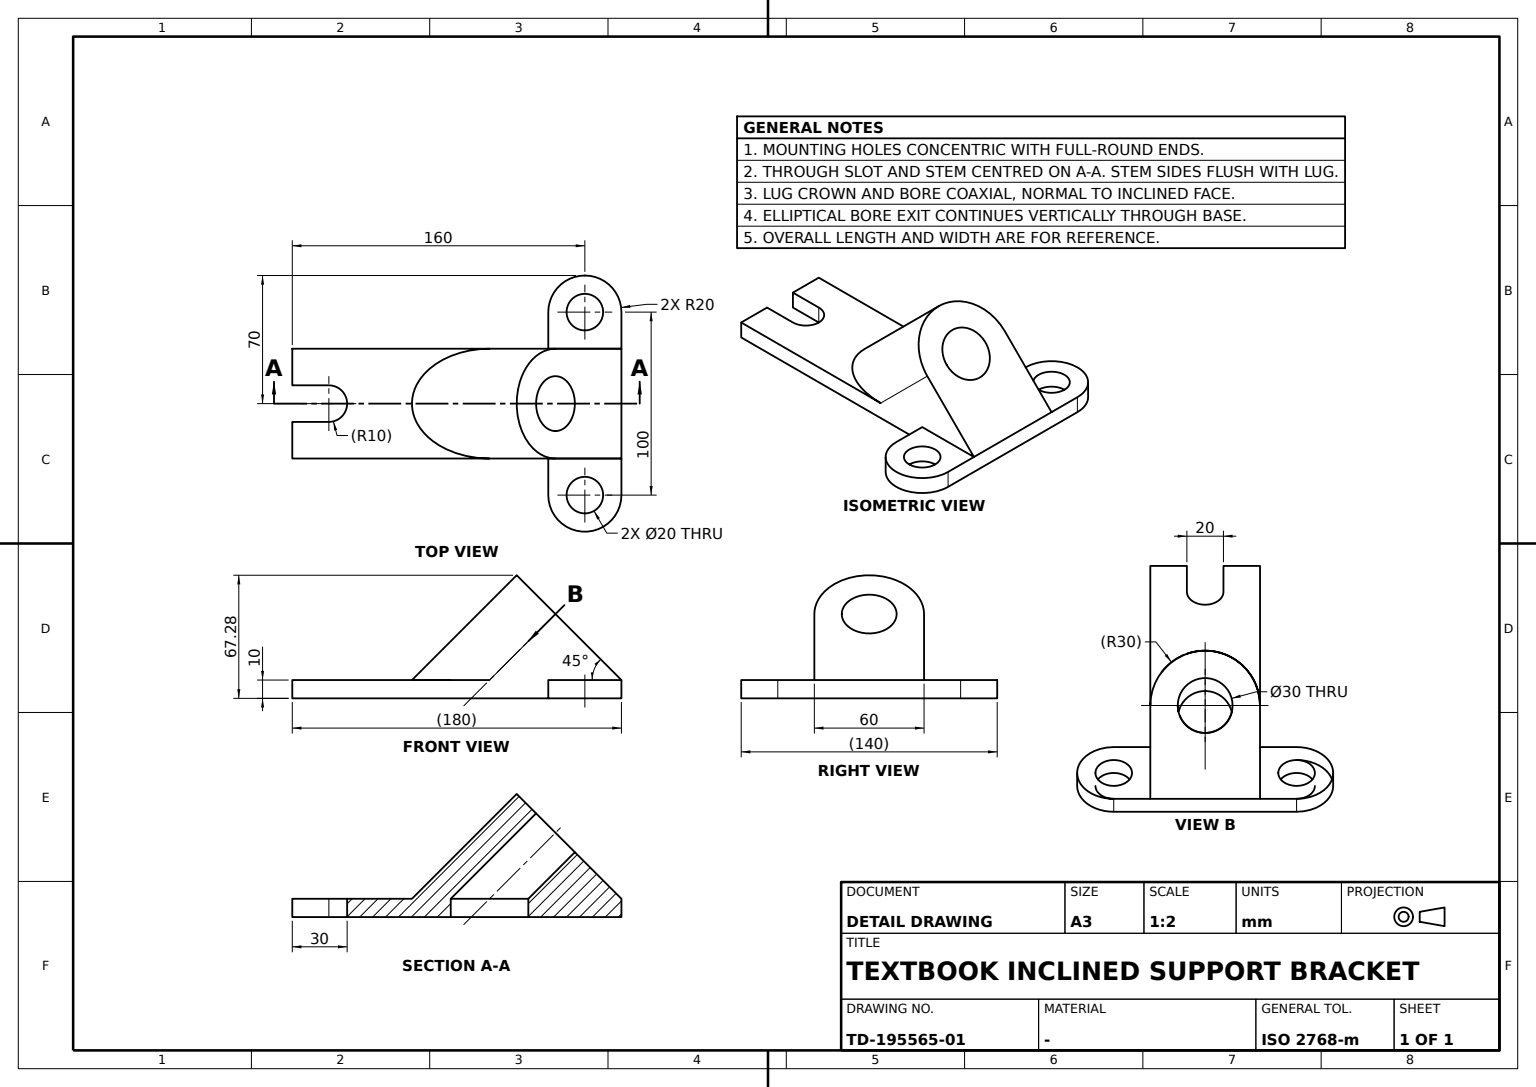
ISO-10303-21;
HEADER;
FILE_DESCRIPTION((''),'2;1');
FILE_NAME('','',(''),(''),'','','');
FILE_SCHEMA(('AUTOMOTIVE_DESIGN'));
ENDSEC;
DATA;
#1=APPLICATION_CONTEXT('');
#2=PRODUCT_CONTEXT('',#1,'mechanical');
#3=PRODUCT('','','',(#2));
#4=PRODUCT_DEFINITION_FORMATION('','',#3);
#5=PRODUCT_DEFINITION_CONTEXT('',#1,'design');
#6=PRODUCT_DEFINITION('','',#4,#5);
#7=PRODUCT_DEFINITION_SHAPE('','',#6);
#8=(LENGTH_UNIT()NAMED_UNIT(*)SI_UNIT(.MILLI.,.METRE.));
#9=(NAMED_UNIT(*)PLANE_ANGLE_UNIT()SI_UNIT($,.RADIAN.));
#10=(NAMED_UNIT(*)SI_UNIT($,.STERADIAN.)SOLID_ANGLE_UNIT());
#11=UNCERTAINTY_MEASURE_WITH_UNIT(LENGTH_MEASURE(1.E-05),#8,'distance_accuracy_value','');
#12=(GEOMETRIC_REPRESENTATION_CONTEXT(3)GLOBAL_UNCERTAINTY_ASSIGNED_CONTEXT((#11))GLOBAL_UNIT_ASSIGNED_CONTEXT((#8,#9,#10))REPRESENTATION_CONTEXT('',''));
#13=CARTESIAN_POINT('',(20.,50.,0.));
#14=VERTEX_POINT('',#13);
#15=CARTESIAN_POINT('',(20.,50.,-10.));
#16=VERTEX_POINT('',#15);
#17=CARTESIAN_POINT('',(20.,50.,-5.));
#18=DIRECTION('',(0.,0.,-1.));
#19=VECTOR('',#18,1000.);
#20=LINE('',#17,#19);
#21=EDGE_CURVE('',#14,#16,#20,.T.);
#22=ORIENTED_EDGE('',*,*,#21,.T.);
#23=CARTESIAN_POINT('',(0.,70.,-10.));
#24=VERTEX_POINT('',#23);
#25=CARTESIAN_POINT('',(0.,50.,-10.));
#26=DIRECTION('',(0.,0.,1.));
#27=DIRECTION('',(0.,1.,0.));
#28=AXIS2_PLACEMENT_3D('',#25,#26,#27);
#29=CIRCLE('',#28,20.);
#30=EDGE_CURVE('',#16,#24,#29,.T.);
#31=ORIENTED_EDGE('',*,*,#30,.T.);
#32=CARTESIAN_POINT('',(0.,70.,0.));
#33=VERTEX_POINT('',#32);
#34=CARTESIAN_POINT('',(0.,70.,-5.));
#35=LINE('',#34,#19);
#36=EDGE_CURVE('',#33,#24,#35,.T.);
#37=ORIENTED_EDGE('',*,*,#36,.F.);
#38=CARTESIAN_POINT('',(0.,50.,0.));
#39=AXIS2_PLACEMENT_3D('',#38,#26,#27);
#40=CIRCLE('',#39,20.);
#41=EDGE_CURVE('',#14,#33,#40,.T.);
#42=ORIENTED_EDGE('',*,*,#41,.F.);
#43=EDGE_LOOP('',(#22,#31,#37,#42));
#44=FACE_OUTER_BOUND('',#43,.T.);
#45=CARTESIAN_POINT('',(0.,50.,-5.));
#46=AXIS2_PLACEMENT_3D('',#45,#18,#27);
#47=CYLINDRICAL_SURFACE('',#46,20.);
#48=ADVANCED_FACE('',(#44),#47,.T.);
#49=ORIENTED_EDGE('',*,*,#36,.T.);
#50=CARTESIAN_POINT('',(-20.,50.,-10.));
#51=VERTEX_POINT('',#50);
#52=EDGE_CURVE('',#24,#51,#29,.T.);
#53=ORIENTED_EDGE('',*,*,#52,.T.);
#54=CARTESIAN_POINT('',(-20.,50.,0.));
#55=VERTEX_POINT('',#54);
#56=CARTESIAN_POINT('',(-20.,50.,-5.));
#57=LINE('',#56,#19);
#58=EDGE_CURVE('',#55,#51,#57,.T.);
#59=ORIENTED_EDGE('',*,*,#58,.F.);
#60=EDGE_CURVE('',#33,#55,#40,.T.);
#61=ORIENTED_EDGE('',*,*,#60,.F.);
#62=EDGE_LOOP('',(#49,#53,#59,#61));
#63=FACE_OUTER_BOUND('',#62,.T.);
#64=ADVANCED_FACE('',(#63),#47,.T.);
#65=CARTESIAN_POINT('',(-20.,-30.,0.));
#66=VERTEX_POINT('',#65);
#67=CARTESIAN_POINT('',(-20.,-50.,0.));
#68=VERTEX_POINT('',#67);
#69=CARTESIAN_POINT('',(-20.,-40.,0.));
#70=DIRECTION('',(0.,-1.,0.));
#71=VECTOR('',#70,1000.);
#72=LINE('',#69,#71);
#73=EDGE_CURVE('',#66,#68,#72,.T.);
#74=ORIENTED_EDGE('',*,*,#73,.F.);
#75=CARTESIAN_POINT('',(-20.,-30.,-10.));
#76=VERTEX_POINT('',#75);
#77=CARTESIAN_POINT('',(-20.,-30.,-5.));
#78=LINE('',#77,#19);
#79=EDGE_CURVE('',#66,#76,#78,.T.);
#80=ORIENTED_EDGE('',*,*,#79,.T.);
#81=CARTESIAN_POINT('',(-20.,-50.,-10.));
#82=VERTEX_POINT('',#81);
#83=CARTESIAN_POINT('',(-20.,-40.,-10.));
#84=LINE('',#83,#71);
#85=EDGE_CURVE('',#76,#82,#84,.T.);
#86=ORIENTED_EDGE('',*,*,#85,.T.);
#87=CARTESIAN_POINT('',(-20.,-50.,-5.));
#88=LINE('',#87,#19);
#89=EDGE_CURVE('',#68,#82,#88,.T.);
#90=ORIENTED_EDGE('',*,*,#89,.F.);
#91=EDGE_LOOP('',(#74,#80,#86,#90));
#92=FACE_OUTER_BOUND('',#91,.T.);
#93=CARTESIAN_POINT('',(-20.,30.,0.));
#94=DIRECTION('',(-1.,0.,0.));
#95=AXIS2_PLACEMENT_3D('',#93,#94,#27);
#96=PLANE('',#95);
#97=ADVANCED_FACE('',(#92),#96,.T.);
#98=CARTESIAN_POINT('',(0.,60.,-10.));
#99=VERTEX_POINT('',#98);
#100=CARTESIAN_POINT('',(0.,40.,-10.));
#101=VERTEX_POINT('',#100);
#102=CIRCLE('',#28,10.);
#103=EDGE_CURVE('',#99,#101,#102,.T.);
#104=ORIENTED_EDGE('',*,*,#103,.T.);
#105=EDGE_CURVE('',#101,#99,#102,.T.);
#106=ORIENTED_EDGE('',*,*,#105,.T.);
#107=EDGE_LOOP('',(#104,#106));
#108=FACE_BOUND('',#107,.T.);
#109=CARTESIAN_POINT('',(-52.1249,-15.,-10.));
#110=VERTEX_POINT('',#109);
#111=CARTESIAN_POINT('',(-52.124884,15.,-10.));
#112=VERTEX_POINT('',#111);
#113=CARTESIAN_POINT('',(-51.464255,-15.,-10.));
#114=CARTESIAN_POINT('',(-50.4775,-14.967538,-10.));
#115=CARTESIAN_POINT('',(-49.333657,-14.872855,-10.));
#116=CARTESIAN_POINT('',(-48.845018,-14.820103,-10.));
#117=CARTESIAN_POINT('',(-48.519609,-14.78223,-10.));
#118=CARTESIAN_POINT('',(-48.358208,-14.762091,-10.));
#119=CARTESIAN_POINT('',(-47.540806,-14.65313,-10.));
#120=CARTESIAN_POINT('',(-46.57273,-14.490561,-10.));
#121=CARTESIAN_POINT('',(-45.465718,-14.245219,-10.));
#122=CARTESIAN_POINT('',(-44.996087,-14.128141,-10.));
#123=CARTESIAN_POINT('',(-44.684066,-14.047437,-10.));
#124=CARTESIAN_POINT('',(-44.530553,-14.006305,-10.));
#125=CARTESIAN_POINT('',(-43.746021,-13.788565,-10.));
#126=CARTESIAN_POINT('',(-42.826179,-13.496945,-10.));
#127=CARTESIAN_POINT('',(-41.790825,-13.10364,-10.));
#128=CARTESIAN_POINT('',(-41.282596,-12.893718,-10.));
#129=CARTESIAN_POINT('',(-41.066809,-12.800907,-10.));
#130=CARTESIAN_POINT('',(-40.9234,-12.738402,-10.));
#131=CARTESIAN_POINT('',(-40.853165,-12.707389,-10.));
#132=CARTESIAN_POINT('',(-40.200687,-12.41542,-10.));
#133=CARTESIAN_POINT('',(-39.361148,-11.998288,-10.));
#134=CARTESIAN_POINT('',(-38.434944,-11.462915,-10.));
#135=CARTESIAN_POINT('',(-37.985157,-11.183048,-10.));
#136=CARTESIAN_POINT('',(-37.795243,-11.060495,-10.));
#137=CARTESIAN_POINT('',(-37.669269,-10.978213,-10.));
#138=CARTESIAN_POINT('',(-37.607907,-10.937658,-10.));
#139=CARTESIAN_POINT('',(-37.034946,-10.554288,-10.));
#140=CARTESIAN_POINT('',(-36.310126,-10.018991,-10.));
#141=CARTESIAN_POINT('',(-35.532976,-9.35224,-10.));
#142=CARTESIAN_POINT('',(-35.16152,-9.008305,-10.));
#143=CARTESIAN_POINT('',(-35.005993,-8.858641,-10.));
#144=CARTESIAN_POINT('',(-34.903123,-8.758363,-10.));
#145=CARTESIAN_POINT('',(-34.853167,-8.709044,-10.));
#146=CARTESIAN_POINT('',(-34.387949,-8.243621,-10.));
#147=CARTESIAN_POINT('',(-33.814771,-7.60411,-10.));
#148=CARTESIAN_POINT('',(-33.228508,-6.824857,-10.));
#149=CARTESIAN_POINT('',(-32.955987,-6.426941,-10.));
#150=CARTESIAN_POINT('',(-32.843609,-6.254629,-10.));
#151=CARTESIAN_POINT('',(-32.769672,-6.13936,-10.));
#152=CARTESIAN_POINT('',(-32.733816,-6.08253,-10.));
#153=CARTESIAN_POINT('',(-32.404339,-5.551247,-10.));
#154=CARTESIAN_POINT('',(-32.018446,-4.830623,-10.));
#155=CARTESIAN_POINT('',(-31.661704,-3.968463,-10.));
#156=CARTESIAN_POINT('',(-31.528842,-3.594373,-10.));
#157=CARTESIAN_POINT('',(-31.444719,-3.343959,-10.));
#158=CARTESIAN_POINT('',(-31.405233,-3.21942,-10.));
#159=CARTESIAN_POINT('',(-31.063576,-2.072772,-10.));
#160=CARTESIAN_POINT('',(-30.911717,-1.041455,-10.));
#161=CARTESIAN_POINT('',(-30.911684,0.521214,-10.));
#162=CARTESIAN_POINT('',(-30.968662,1.298476,-10.));
#163=CARTESIAN_POINT('',(-31.134877,2.198154,-10.));
#164=CARTESIAN_POINT('',(-31.227486,2.582202,-10.));
#165=CARTESIAN_POINT('',(-31.293974,2.837895,-10.));
#166=CARTESIAN_POINT('',(-31.330001,2.966942,-10.));
#167=CARTESIAN_POINT('',(-31.517929,3.59763,-10.));
#168=CARTESIAN_POINT('',(-31.796954,4.342448,-10.));
#169=CARTESIAN_POINT('',(-32.21613,5.190392,-10.));
#170=CARTESIAN_POINT('',(-32.449129,5.609112,-10.));
#171=CARTESIAN_POINT('',(-32.554002,5.787437,-10.));
#172=CARTESIAN_POINT('',(-32.625033,5.906071,-10.));
#173=CARTESIAN_POINT('',(-32.661773,5.966339,-10.));
#174=CARTESIAN_POINT('',(-32.985436,6.488252,-10.));
#175=CARTESIAN_POINT('',(-33.464246,7.165387,-10.));
#176=CARTESIAN_POINT('',(-34.105562,7.922569,-10.));
#177=CARTESIAN_POINT('',(-34.446896,8.292957,-10.));
#178=CARTESIAN_POINT('',(-34.597613,8.449938,-10.));
#179=CARTESIAN_POINT('',(-34.699075,8.554201,-10.));
#180=CARTESIAN_POINT('',(-34.75143,8.607269,-10.));
#181=CARTESIAN_POINT('',(-35.206692,9.062753,-10.));
#182=CARTESIAN_POINT('',(-35.85305,9.646104,-10.));
#183=CARTESIAN_POINT('',(-36.675981,10.284751,-10.));
#184=CARTESIAN_POINT('',(-37.104659,10.593591,-10.));
#185=CARTESIAN_POINT('',(-37.292066,10.723705,-10.));
#186=CARTESIAN_POINT('',(-37.417824,10.809948,-10.));
#187=CARTESIAN_POINT('',(-37.482477,10.853733,-10.));
#188=CARTESIAN_POINT('',(-38.043479,11.229116,-10.));
#189=CARTESIAN_POINT('',(-38.822157,11.701895,-10.));
#190=CARTESIAN_POINT('',(-39.784298,12.204942,-10.));
#191=CARTESIAN_POINT('',(-40.278789,12.444333,-10.));
#192=CARTESIAN_POINT('',(-40.49359,12.544329,-10.));
#193=CARTESIAN_POINT('',(-40.63743,12.610416,-10.));
#194=CARTESIAN_POINT('',(-40.711009,12.64377,-10.));
#195=CARTESIAN_POINT('',(-41.351977,12.930563,-10.));
#196=CARTESIAN_POINT('',(-42.228444,13.282712,-10.));
#197=CARTESIAN_POINT('',(-43.289218,13.640628,-10.));
#198=CARTESIAN_POINT('',(-43.829161,13.806355,-10.));
#199=CARTESIAN_POINT('',(-44.062613,13.874546,-10.));
#200=CARTESIAN_POINT('',(-44.218703,13.919377,-10.));
#201=CARTESIAN_POINT('',(-44.298075,13.941782,-10.));
#202=CARTESIAN_POINT('',(-44.994684,14.135104,-10.));
#203=CARTESIAN_POINT('',(-45.936536,14.361122,-10.));
#204=CARTESIAN_POINT('',(-47.058182,14.569257,-10.));
#205=CARTESIAN_POINT('',(-47.543777,14.646554,-10.));
#206=CARTESIAN_POINT('',(-47.868594,14.695439,-10.));
#207=CARTESIAN_POINT('',(-48.032751,14.71872,-10.));
#208=CARTESIAN_POINT('',(-49.493363,14.913453,-10.));
#209=CARTESIAN_POINT('',(-50.803311,14.999997,-10.));
#210=B_SPLINE_CURVE_WITH_KNOTS('',3,(#109,#113,#114,#115,#116,#117,#118,#119,#120,#121,#122,#123,#124,#125,#126,#127,#128,#129,#130,#131,#132,#133,#134,#135,#136,#137,#138,#139,#140,#141,#142,#143,#144,#145,#146,#147,#148,#149,#150,#151,#152,#153,#154,#155,#156,#157,#158,#159,#160,#161,#162,#163,#164,#165,#166,#167,#168,#169,#170,#171,#172,#173,#174,#175,#176,#177,#178,#179,#180,#181,#182,#183,#184,#185,#186,#187,#188,#189,#190,#191,#192,#193,#194,#195,#196,#197,#198,#199,#200,#201,#202,#203,#204,#205,#206,#207,#208,#209,#111),.UNSPECIFIED.,.F.,.F.,(4,1,1,2,2,1,1,2,2,1,1,1,2,2,1,1,1,2,2,1,1,1,2,2,1,1,1,2,2,1,1,2,2,2,1,1,2,2,1,1,1,2,2,1,1,1,2,2,1,1,1,2,2,1,1,1,2,2,1,1,1,2,2,1,1,2,2,4),(0.,0.03125,0.046875,0.0546875,0.0625,0.09375,0.109375,0.1171875,0.125,0.15625,0.171875,0.1796875,0.18359375,0.1875,0.21875,0.234375,0.2421875,0.24609375,0.25,0.28125,0.296875,0.3046875,0.30859375,0.3125,0.34375,0.359375,0.3671875,0.37109375,0.375,0.40625,0.421875,0.4296875,0.4375,0.5,0.53125,0.546875,0.5546875,0.5625,0.59375,0.609375,0.6171875,0.62109375,0.625,0.65625,0.671875,0.6796875,0.68359375,0.6875,0.71875,0.734375,0.7421875,0.74609375,0.75,0.78125,0.796875,0.8046875,0.80859375,0.8125,0.84375,0.859375,0.8671875,0.87109375,0.875,0.90625,0.921875,0.9296875,0.9375,1.),.UNSPECIFIED.);
#211=EDGE_CURVE('',#110,#112,#210,.T.);
#212=ORIENTED_EDGE('',*,*,#211,.T.);
#213=CARTESIAN_POINT('',(-52.785777,14.999988,-10.));
#214=CARTESIAN_POINT('',(-53.772897,14.9675,-10.));
#215=CARTESIAN_POINT('',(-54.753686,14.886288,-10.));
#216=CARTESIAN_POINT('',(-55.406139,14.821318,-10.));
#217=CARTESIAN_POINT('',(-55.729535,14.783704,-10.));
#218=CARTESIAN_POINT('',(-56.710377,14.652915,-10.));
#219=CARTESIAN_POINT('',(-57.678403,14.490313,-10.));
#220=CARTESIAN_POINT('',(-58.785341,14.244935,-10.));
#221=CARTESIAN_POINT('',(-59.254938,14.127843,-10.));
#222=CARTESIAN_POINT('',(-59.566935,14.04713,-10.));
#223=CARTESIAN_POINT('',(-59.720493,14.005977,-10.));
#224=CARTESIAN_POINT('',(-60.504673,13.788294,-10.));
#225=CARTESIAN_POINT('',(-61.424119,13.496763,-10.));
#226=CARTESIAN_POINT('',(-62.459062,13.103599,-10.));
#227=CARTESIAN_POINT('',(-62.967096,12.893755,-10.));
#228=CARTESIAN_POINT('',(-63.182803,12.80098,-10.));
#229=CARTESIAN_POINT('',(-63.326159,12.738499,-10.));
#230=CARTESIAN_POINT('',(-63.396345,12.70751,-10.));
#231=CARTESIAN_POINT('',(-64.048804,12.415558,-10.));
#232=CARTESIAN_POINT('',(-64.888319,11.998449,-10.));
#233=CARTESIAN_POINT('',(-65.814499,11.463106,-10.));
#234=CARTESIAN_POINT('',(-66.264276,11.183255,-10.));
#235=CARTESIAN_POINT('',(-66.454184,11.060708,-10.));
#236=CARTESIAN_POINT('',(-66.580156,10.978431,-10.));
#237=CARTESIAN_POINT('',(-66.641495,10.937892,-10.));
#238=CARTESIAN_POINT('',(-67.21463,10.554417,-10.));
#239=CARTESIAN_POINT('',(-67.93965,10.018983,-10.));
#240=CARTESIAN_POINT('',(-68.716978,9.352079,-10.));
#241=CARTESIAN_POINT('',(-69.088509,9.008068,-10.));
#242=CARTESIAN_POINT('',(-69.244066,8.858373,-10.));
#243=CARTESIAN_POINT('',(-69.346954,8.758073,-10.));
#244=CARTESIAN_POINT('',(-69.396928,8.708735,-10.));
#245=CARTESIAN_POINT('',(-69.86215,8.243291,-10.));
#246=CARTESIAN_POINT('',(-70.435334,7.603739,-10.));
#247=CARTESIAN_POINT('',(-71.021601,6.824415,-10.));
#248=CARTESIAN_POINT('',(-71.294123,6.426458,-10.));
#249=CARTESIAN_POINT('',(-71.406501,6.254128,-10.));
#250=CARTESIAN_POINT('',(-71.480438,6.138846,-10.));
#251=CARTESIAN_POINT('',(-71.516301,6.082001,-10.));
#252=CARTESIAN_POINT('',(-71.845728,5.550738,-10.));
#253=CARTESIAN_POINT('',(-72.23156,4.830146,-10.));
#254=CARTESIAN_POINT('',(-72.588241,3.96803,-10.));
#255=CARTESIAN_POINT('',(-72.721077,3.593961,-10.));
#256=CARTESIAN_POINT('',(-72.805184,3.343561,-10.));
#257=CARTESIAN_POINT('',(-72.844667,3.219014,-10.));
#258=CARTESIAN_POINT('',(-73.186211,2.072576,-10.));
#259=CARTESIAN_POINT('',(-73.338033,1.041624,-10.));
#260=CARTESIAN_POINT('',(-73.338106,-0.520967,-10.));
#261=CARTESIAN_POINT('',(-73.281152,-1.298191,-10.));
#262=CARTESIAN_POINT('',(-73.114973,-2.197829,-10.));
#263=CARTESIAN_POINT('',(-73.022382,-2.581862,-10.));
#264=CARTESIAN_POINT('',(-72.955905,-2.837544,-10.));
#265=CARTESIAN_POINT('',(-72.919887,-2.966577,-10.));
#266=CARTESIAN_POINT('',(-72.731976,-3.597282,-10.));
#267=CARTESIAN_POINT('',(-72.45297,-4.342121,-10.));
#268=CARTESIAN_POINT('',(-72.033814,-5.190088,-10.));
#269=CARTESIAN_POINT('',(-71.800823,-5.608818,-10.));
#270=CARTESIAN_POINT('',(-71.695953,-5.787148,-10.));
#271=CARTESIAN_POINT('',(-71.624925,-5.905785,-10.));
#272=CARTESIAN_POINT('',(-71.588186,-5.966055,-10.));
#273=CARTESIAN_POINT('',(-71.264534,-6.487978,-10.));
#274=CARTESIAN_POINT('',(-70.785736,-7.165129,-10.));
#275=CARTESIAN_POINT('',(-70.144428,-7.922333,-10.));
#276=CARTESIAN_POINT('',(-69.803096,-8.292733,-10.));
#277=CARTESIAN_POINT('',(-69.65238,-8.449719,-10.));
#278=CARTESIAN_POINT('',(-69.550919,-8.553985,-10.));
#279=CARTESIAN_POINT('',(-69.498564,-8.607055,-10.));
#280=CARTESIAN_POINT('',(-69.04331,-9.062548,-10.));
#281=CARTESIAN_POINT('',(-68.396962,-9.645911,-10.));
#282=CARTESIAN_POINT('',(-67.57404,-10.284571,-10.));
#283=CARTESIAN_POINT('',(-67.145367,-10.593418,-10.));
#284=CARTESIAN_POINT('',(-66.957962,-10.723535,-10.));
#285=CARTESIAN_POINT('',(-66.832205,-10.80978,-10.));
#286=CARTESIAN_POINT('',(-66.767551,-10.853567,-10.));
#287=CARTESIAN_POINT('',(-66.206564,-11.228953,-10.));
#288=CARTESIAN_POINT('',(-65.427906,-11.701736,-10.));
#289=CARTESIAN_POINT('',(-64.465789,-12.204789,-10.));
#290=CARTESIAN_POINT('',(-63.971311,-12.444183,-10.));
#291=CARTESIAN_POINT('',(-63.756516,-12.544181,-10.));
#292=CARTESIAN_POINT('',(-63.61268,-12.610269,-10.));
#293=CARTESIAN_POINT('',(-63.539104,-12.643623,-10.));
#294=CARTESIAN_POINT('',(-62.898138,-12.930427,-10.));
#295=CARTESIAN_POINT('',(-62.021669,-13.28259,-10.));
#296=CARTESIAN_POINT('',(-60.96089,-13.640524,-10.));
#297=CARTESIAN_POINT('',(-60.420942,-13.806259,-10.));
#298=CARTESIAN_POINT('',(-60.187487,-13.874454,-10.));
#299=CARTESIAN_POINT('',(-60.031396,-13.919286,-10.));
#300=CARTESIAN_POINT('',(-59.952025,-13.941692,-10.));
#301=CARTESIAN_POINT('',(-59.255395,-14.135029,-10.));
#302=CARTESIAN_POINT('',(-58.313513,-14.361064,-10.));
#303=CARTESIAN_POINT('',(-57.191829,-14.569217,-10.));
#304=CARTESIAN_POINT('',(-56.706218,-14.64652,-10.));
#305=CARTESIAN_POINT('',(-56.38139,-14.69541,-10.));
#306=CARTESIAN_POINT('',(-56.217229,-14.718693,-10.));
#307=CARTESIAN_POINT('',(-54.756558,-14.913444,-10.));
#308=CARTESIAN_POINT('',(-53.446547,-15.,-10.));
#309=B_SPLINE_CURVE_WITH_KNOTS('',3,(#111,#213,#214,#215,#216,#217,#218,#219,#220,#221,#222,#223,#224,#225,#226,#227,#228,#229,#230,#231,#232,#233,#234,#235,#236,#237,#238,#239,#240,#241,#242,#243,#244,#245,#246,#247,#248,#249,#250,#251,#252,#253,#254,#255,#256,#257,#258,#259,#260,#261,#262,#263,#264,#265,#266,#267,#268,#269,#270,#271,#272,#273,#274,#275,#276,#277,#278,#279,#280,#281,#282,#283,#284,#285,#286,#287,#288,#289,#290,#291,#292,#293,#294,#295,#296,#297,#298,#299,#300,#301,#302,#303,#304,#305,#306,#307,#308,#109),.UNSPECIFIED.,.F.,.F.,(4,1,2,2,1,1,2,2,1,1,1,2,2,1,1,1,2,2,1,1,1,2,2,1,1,1,2,2,1,1,2,2,2,1,1,2,2,1,1,1,2,2,1,1,1,2,2,1,1,1,2,2,1,1,1,2,2,1,1,1,2,2,1,1,2,2,4),(0.,0.03125,0.046875,0.0625,0.09375,0.109375,0.1171875,0.125,0.15625,0.171875,0.1796875,0.18359375,0.1875,0.21875,0.234375,0.2421875,0.24609375,0.25,0.28125,0.296875,0.3046875,0.30859375,0.3125,0.34375,0.359375,0.3671875,0.37109375,0.375,0.40625,0.421875,0.4296875,0.4375,0.5,0.53125,0.546875,0.5546875,0.5625,0.59375,0.609375,0.6171875,0.62109375,0.625,0.65625,0.671875,0.6796875,0.68359375,0.6875,0.71875,0.734375,0.7421875,0.74609375,0.75,0.78125,0.796875,0.8046875,0.80859375,0.8125,0.84375,0.859375,0.8671875,0.87109375,0.875,0.90625,0.921875,0.9296875,0.9375,1.),.UNSPECIFIED.);
#310=EDGE_CURVE('',#112,#110,#309,.T.);
#311=ORIENTED_EDGE('',*,*,#310,.T.);
#312=EDGE_LOOP('',(#212,#311));
#313=FACE_BOUND('',#312,.T.);
#314=CARTESIAN_POINT('',(0.,-60.,-10.));
#315=VERTEX_POINT('',#314);
#316=CARTESIAN_POINT('',(0.,-40.,-10.));
#317=VERTEX_POINT('',#316);
#318=CARTESIAN_POINT('',(0.,-50.,-10.));
#319=AXIS2_PLACEMENT_3D('',#318,#26,#27);
#320=CIRCLE('',#319,10.);
#321=EDGE_CURVE('',#315,#317,#320,.T.);
#322=ORIENTED_EDGE('',*,*,#321,.T.);
#323=EDGE_CURVE('',#317,#315,#320,.T.);
#324=ORIENTED_EDGE('',*,*,#323,.T.);
#325=EDGE_LOOP('',(#322,#324));
#326=FACE_BOUND('',#325,.T.);
#327=CARTESIAN_POINT('',(-20.,30.,-10.));
#328=VERTEX_POINT('',#327);
#329=CARTESIAN_POINT('',(-159.999708,30.,-10.));
#330=VERTEX_POINT('',#329);
#331=CARTESIAN_POINT('',(-89.999854,30.,-10.));
#332=VECTOR('',#94,1000.);
#333=LINE('',#331,#332);
#334=EDGE_CURVE('',#328,#330,#333,.T.);
#335=ORIENTED_EDGE('',*,*,#334,.F.);
#336=CARTESIAN_POINT('',(-20.,40.,-10.));
#337=LINE('',#336,#71);
#338=EDGE_CURVE('',#51,#328,#337,.T.);
#339=ORIENTED_EDGE('',*,*,#338,.F.);
#340=ORIENTED_EDGE('',*,*,#52,.F.);
#341=ORIENTED_EDGE('',*,*,#30,.F.);
#342=CARTESIAN_POINT('',(20.,-50.,-10.));
#343=VERTEX_POINT('',#342);
#344=CARTESIAN_POINT('',(20.,0.,-10.));
#345=VECTOR('',#27,1000.);
#346=LINE('',#344,#345);
#347=EDGE_CURVE('',#343,#16,#346,.T.);
#348=ORIENTED_EDGE('',*,*,#347,.F.);
#349=CIRCLE('',#319,20.);
#350=EDGE_CURVE('',#82,#343,#349,.T.);
#351=ORIENTED_EDGE('',*,*,#350,.F.);
#352=ORIENTED_EDGE('',*,*,#85,.F.);
#353=CARTESIAN_POINT('',(-159.999708,-30.,-10.));
#354=VERTEX_POINT('',#353);
#355=CARTESIAN_POINT('',(-89.999854,-30.,-10.));
#356=DIRECTION('',(1.,0.,0.));
#357=VECTOR('',#356,1000.);
#358=LINE('',#355,#357);
#359=EDGE_CURVE('',#354,#76,#358,.T.);
#360=ORIENTED_EDGE('',*,*,#359,.F.);
#361=CARTESIAN_POINT('',(-159.999708,-10.,-10.));
#362=VERTEX_POINT('',#361);
#363=CARTESIAN_POINT('',(-159.999708,-20.,-10.));
#364=LINE('',#363,#71);
#365=EDGE_CURVE('',#362,#354,#364,.T.);
#366=ORIENTED_EDGE('',*,*,#365,.F.);
#367=CARTESIAN_POINT('',(-139.999708,-10.,-10.));
#368=VERTEX_POINT('',#367);
#369=CARTESIAN_POINT('',(-149.999708,-10.,-10.));
#370=LINE('',#369,#357);
#371=EDGE_CURVE('',#362,#368,#370,.T.);
#372=ORIENTED_EDGE('',*,*,#371,.T.);
#373=CARTESIAN_POINT('',(-139.999708,10.,-10.));
#374=VERTEX_POINT('',#373);
#375=CARTESIAN_POINT('',(-139.999708,0.,-10.));
#376=AXIS2_PLACEMENT_3D('',#375,#26,#27);
#377=CIRCLE('',#376,10.);
#378=EDGE_CURVE('',#368,#374,#377,.T.);
#379=ORIENTED_EDGE('',*,*,#378,.T.);
#380=CARTESIAN_POINT('',(-159.999708,10.,-10.));
#381=VERTEX_POINT('',#380);
#382=CARTESIAN_POINT('',(-149.999708,10.,-10.));
#383=LINE('',#382,#332);
#384=EDGE_CURVE('',#374,#381,#383,.T.);
#385=ORIENTED_EDGE('',*,*,#384,.T.);
#386=CARTESIAN_POINT('',(-159.999708,20.,-10.));
#387=LINE('',#386,#71);
#388=EDGE_CURVE('',#330,#381,#387,.T.);
#389=ORIENTED_EDGE('',*,*,#388,.F.);
#390=EDGE_LOOP('',(#335,#339,#340,#341,#348,#351,#352,#360,#366,#372,#379,#385,#389));
#391=FACE_OUTER_BOUND('',#390,.T.);
#392=CARTESIAN_POINT('',(0.,0.,-10.));
#393=AXIS2_PLACEMENT_3D('',#392,#26,#27);
#394=PLANE('',#393);
#395=ADVANCED_FACE('',(#108,#313,#326,#391),#394,.F.);
#396=CARTESIAN_POINT('',(-139.999708,-10.,0.));
#397=VERTEX_POINT('',#396);
#398=CARTESIAN_POINT('',(-139.999708,-10.,-5.));
#399=LINE('',#398,#19);
#400=EDGE_CURVE('',#397,#368,#399,.T.);
#401=ORIENTED_EDGE('',*,*,#400,.F.);
#402=CARTESIAN_POINT('',(-139.999708,10.,0.));
#403=VERTEX_POINT('',#402);
#404=CARTESIAN_POINT('',(-139.999708,0.,0.));
#405=AXIS2_PLACEMENT_3D('',#404,#26,#27);
#406=CIRCLE('',#405,10.);
#407=EDGE_CURVE('',#397,#403,#406,.T.);
#408=ORIENTED_EDGE('',*,*,#407,.T.);
#409=CARTESIAN_POINT('',(-139.999708,10.,-5.));
#410=LINE('',#409,#19);
#411=EDGE_CURVE('',#403,#374,#410,.T.);
#412=ORIENTED_EDGE('',*,*,#411,.T.);
#413=ORIENTED_EDGE('',*,*,#378,.F.);
#414=EDGE_LOOP('',(#401,#408,#412,#413));
#415=FACE_OUTER_BOUND('',#414,.T.);
#416=CARTESIAN_POINT('',(-139.999708,0.,-5.));
#417=AXIS2_PLACEMENT_3D('',#416,#18,#27);
#418=CYLINDRICAL_SURFACE('',#417,10.);
#419=ADVANCED_FACE('',(#415),#418,.F.);
#420=CARTESIAN_POINT('',(-159.999708,-10.,0.));
#421=VERTEX_POINT('',#420);
#422=CARTESIAN_POINT('',(-149.999708,-10.,0.));
#423=LINE('',#422,#357);
#424=EDGE_CURVE('',#421,#397,#423,.T.);
#425=ORIENTED_EDGE('',*,*,#424,.F.);
#426=CARTESIAN_POINT('',(-159.999708,-30.,0.));
#427=VERTEX_POINT('',#426);
#428=CARTESIAN_POINT('',(-159.999708,-20.,0.));
#429=LINE('',#428,#71);
#430=EDGE_CURVE('',#421,#427,#429,.T.);
#431=ORIENTED_EDGE('',*,*,#430,.T.);
#432=CARTESIAN_POINT('',(-52.124892,-30.,0.));
#433=VERTEX_POINT('',#432);
#434=CARTESIAN_POINT('',(-106.0623,-30.,0.));
#435=LINE('',#434,#357);
#436=EDGE_CURVE('',#427,#433,#435,.T.);
#437=ORIENTED_EDGE('',*,*,#436,.T.);
#438=CARTESIAN_POINT('',(-52.124892,30.,0.));
#439=VERTEX_POINT('',#438);
#440=CARTESIAN_POINT('',(-55.125369,30.,0.));
#441=CARTESIAN_POINT('',(-58.125846,29.81244,0.));
#442=CARTESIAN_POINT('',(-61.110662,29.437321,0.));
#443=CARTESIAN_POINT('',(-66.743283,28.356856,0.));
#444=CARTESIAN_POINT('',(-72.184496,26.551422,0.));
#445=CARTESIAN_POINT('',(-74.713365,25.522769,0.));
#446=CARTESIAN_POINT('',(-79.216544,23.302689,0.));
#447=CARTESIAN_POINT('',(-83.340082,20.446852,0.));
#448=CARTESIAN_POINT('',(-85.124292,19.005473,0.));
#449=CARTESIAN_POINT('',(-87.94598,16.31053,0.));
#450=CARTESIAN_POINT('',(-90.300587,13.209992,0.));
#451=CARTESIAN_POINT('',(-91.179743,11.863508,0.));
#452=CARTESIAN_POINT('',(-92.638686,9.197936,0.));
#453=CARTESIAN_POINT('',(-93.663535,6.339541,0.));
#454=CARTESIAN_POINT('',(-94.039962,4.957233,0.));
#455=CARTESIAN_POINT('',(-94.551559,2.201809,0.));
#456=CARTESIAN_POINT('',(-94.609298,-0.599308,0.));
#457=CARTESIAN_POINT('',(-94.525967,-1.968667,0.));
#458=CARTESIAN_POINT('',(-94.154209,-4.583152,0.));
#459=CARTESIAN_POINT('',(-93.397722,-7.112102,0.));
#460=CARTESIAN_POINT('',(-92.94943,-8.300984,0.));
#461=CARTESIAN_POINT('',(-91.851529,-10.714644,0.));
#462=CARTESIAN_POINT('',(-90.448061,-12.965541,0.));
#463=CARTESIAN_POINT('',(-89.642449,-14.090338,0.));
#464=CARTESIAN_POINT('',(-87.057711,-17.280741,0.));
#465=CARTESIAN_POINT('',(-83.972737,-20.017792,0.));
#466=CARTESIAN_POINT('',(-81.763613,-21.632478,0.));
#467=CARTESIAN_POINT('',(-77.180091,-24.43313,0.));
#468=CARTESIAN_POINT('',(-72.234823,-26.527601,0.));
#469=CARTESIAN_POINT('',(-69.737963,-27.395842,0.));
#470=CARTESIAN_POINT('',(-64.766409,-28.788789,0.));
#471=CARTESIAN_POINT('',(-59.668925,-29.603805,0.));
#472=CARTESIAN_POINT('',(-57.160413,-29.867935,0.));
#473=CARTESIAN_POINT('',(-54.642652,-30.,0.));
#474=B_SPLINE_CURVE_WITH_KNOTS('',5,(#438,#440,#441,#442,#443,#444,#445,#446,#447,#448,#449,#450,#451,#452,#453,#454,#455,#456,#457,#458,#459,#460,#461,#462,#463,#464,#465,#466,#467,#468,#469,#470,#471,#472,#473,#432),.UNSPECIFIED.,.F.,.F.,(6,3,3,3,3,3,3,3,3,3,3,6),(0.,21.216579279,40.459374465,56.60389594,67.929780791,78.017290486,87.677943711,96.634362046,106.391148727,125.62394119,144.26592682,162.069183292),.UNSPECIFIED.);
#475=EDGE_CURVE('',#439,#433,#474,.T.);
#476=ORIENTED_EDGE('',*,*,#475,.F.);
#477=CARTESIAN_POINT('',(-159.999708,30.,0.));
#478=VERTEX_POINT('',#477);
#479=CARTESIAN_POINT('',(-106.0623,30.,0.));
#480=LINE('',#479,#332);
#481=EDGE_CURVE('',#439,#478,#480,.T.);
#482=ORIENTED_EDGE('',*,*,#481,.T.);
#483=CARTESIAN_POINT('',(-159.999708,10.,0.));
#484=VERTEX_POINT('',#483);
#485=CARTESIAN_POINT('',(-159.999708,20.,0.));
#486=LINE('',#485,#71);
#487=EDGE_CURVE('',#478,#484,#486,.T.);
#488=ORIENTED_EDGE('',*,*,#487,.T.);
#489=CARTESIAN_POINT('',(-149.999708,10.,0.));
#490=LINE('',#489,#332);
#491=EDGE_CURVE('',#403,#484,#490,.T.);
#492=ORIENTED_EDGE('',*,*,#491,.F.);
#493=ORIENTED_EDGE('',*,*,#407,.F.);
#494=EDGE_LOOP('',(#425,#431,#437,#476,#482,#488,#492,#493));
#495=FACE_OUTER_BOUND('',#494,.T.);
#496=CARTESIAN_POINT('',(0.,0.,0.));
#497=AXIS2_PLACEMENT_3D('',#496,#26,#27);
#498=PLANE('',#497);
#499=ADVANCED_FACE('',(#495),#498,.T.);
#500=ORIENTED_EDGE('',*,*,#424,.T.);
#501=ORIENTED_EDGE('',*,*,#400,.T.);
#502=ORIENTED_EDGE('',*,*,#371,.F.);
#503=CARTESIAN_POINT('',(-159.999708,-10.,-5.));
#504=LINE('',#503,#19);
#505=EDGE_CURVE('',#421,#362,#504,.T.);
#506=ORIENTED_EDGE('',*,*,#505,.F.);
#507=EDGE_LOOP('',(#500,#501,#502,#506));
#508=FACE_OUTER_BOUND('',#507,.T.);
#509=AXIS2_PLACEMENT_3D('',#396,#70,#94);
#510=PLANE('',#509);
#511=ADVANCED_FACE('',(#508),#510,.F.);
#512=CARTESIAN_POINT('',(-159.999708,10.,-5.));
#513=LINE('',#512,#19);
#514=EDGE_CURVE('',#484,#381,#513,.T.);
#515=ORIENTED_EDGE('',*,*,#514,.T.);
#516=ORIENTED_EDGE('',*,*,#384,.F.);
#517=ORIENTED_EDGE('',*,*,#411,.F.);
#518=ORIENTED_EDGE('',*,*,#491,.T.);
#519=EDGE_LOOP('',(#515,#516,#517,#518));
#520=FACE_OUTER_BOUND('',#519,.T.);
#521=AXIS2_PLACEMENT_3D('',#402,#70,#94);
#522=PLANE('',#521);
#523=ADVANCED_FACE('',(#520),#522,.T.);
#524=CARTESIAN_POINT('',(-16.062446,30.,36.062446));
#525=VERTEX_POINT('',#524);
#526=CARTESIAN_POINT('',(-16.062446,-30.,36.062446));
#527=VERTEX_POINT('',#526);
#528=CARTESIAN_POINT('',(-16.062446,0.,36.062446));
#529=DIRECTION('',(0.707106781,0.,0.707106781));
#530=AXIS2_PLACEMENT_3D('',#528,#529,#27);
#531=CIRCLE('',#530,30.);
#532=EDGE_CURVE('',#525,#527,#531,.T.);
#533=ORIENTED_EDGE('',*,*,#532,.T.);
#534=CARTESIAN_POINT('',(20.,-30.,0.));
#535=VERTEX_POINT('',#534);
#536=CARTESIAN_POINT('',(1.968777,-30.,18.031223));
#537=DIRECTION('',(0.707106781,0.,-0.707106781));
#538=VECTOR('',#537,1000.);
#539=LINE('',#536,#538);
#540=EDGE_CURVE('',#527,#535,#539,.T.);
#541=ORIENTED_EDGE('',*,*,#540,.T.);
#542=CARTESIAN_POINT('',(20.,30.,0.));
#543=VERTEX_POINT('',#542);
#544=CARTESIAN_POINT('',(20.,0.,0.));
#545=LINE('',#544,#345);
#546=EDGE_CURVE('',#535,#543,#545,.T.);
#547=ORIENTED_EDGE('',*,*,#546,.T.);
#548=CARTESIAN_POINT('',(1.968777,30.,18.031223));
#549=DIRECTION('',(-0.707106781,0.,0.707106781));
#550=VECTOR('',#549,1000.);
#551=LINE('',#548,#550);
#552=EDGE_CURVE('',#543,#525,#551,.T.);
#553=ORIENTED_EDGE('',*,*,#552,.T.);
#554=EDGE_LOOP('',(#533,#541,#547,#553));
#555=FACE_OUTER_BOUND('',#554,.T.);
#556=CARTESIAN_POINT('',(-16.062446,-15.,36.062446));
#557=VERTEX_POINT('',#556);
#558=CARTESIAN_POINT('',(-16.062446,15.,36.062446));
#559=VERTEX_POINT('',#558);
#560=CIRCLE('',#530,15.);
#561=EDGE_CURVE('',#557,#559,#560,.T.);
#562=ORIENTED_EDGE('',*,*,#561,.F.);
#563=EDGE_CURVE('',#559,#557,#560,.T.);
#564=ORIENTED_EDGE('',*,*,#563,.F.);
#565=EDGE_LOOP('',(#562,#564));
#566=FACE_BOUND('',#565,.T.);
#567=CARTESIAN_POINT('',(10.,0.,10.));
#568=AXIS2_PLACEMENT_3D('',#567,#529,#27);
#569=PLANE('',#568);
#570=ADVANCED_FACE('',(#555,#566),#569,.T.);
#571=ORIENTED_EDGE('',*,*,#323,.F.);
#572=CARTESIAN_POINT('',(0.,-40.,0.));
#573=VERTEX_POINT('',#572);
#574=CARTESIAN_POINT('',(0.,-40.,-5.));
#575=LINE('',#574,#19);
#576=EDGE_CURVE('',#573,#317,#575,.T.);
#577=ORIENTED_EDGE('',*,*,#576,.F.);
#578=CARTESIAN_POINT('',(0.,-60.,0.));
#579=VERTEX_POINT('',#578);
#580=CARTESIAN_POINT('',(0.,-50.,0.));
#581=AXIS2_PLACEMENT_3D('',#580,#26,#27);
#582=CIRCLE('',#581,10.);
#583=EDGE_CURVE('',#573,#579,#582,.T.);
#584=ORIENTED_EDGE('',*,*,#583,.T.);
#585=CARTESIAN_POINT('',(0.,-60.,-5.));
#586=LINE('',#585,#19);
#587=EDGE_CURVE('',#579,#315,#586,.T.);
#588=ORIENTED_EDGE('',*,*,#587,.T.);
#589=EDGE_LOOP('',(#571,#577,#584,#588));
#590=FACE_OUTER_BOUND('',#589,.T.);
#591=CARTESIAN_POINT('',(0.,-50.,-5.));
#592=AXIS2_PLACEMENT_3D('',#591,#18,#27);
#593=CYLINDRICAL_SURFACE('',#592,10.);
#594=ADVANCED_FACE('',(#590),#593,.F.);
#595=ORIENTED_EDGE('',*,*,#338,.T.);
#596=VERTEX_POINT('',#93);
#597=CARTESIAN_POINT('',(-20.,30.,-5.));
#598=LINE('',#597,#19);
#599=EDGE_CURVE('',#596,#328,#598,.T.);
#600=ORIENTED_EDGE('',*,*,#599,.F.);
#601=CARTESIAN_POINT('',(-20.,40.,0.));
#602=LINE('',#601,#71);
#603=EDGE_CURVE('',#55,#596,#602,.T.);
#604=ORIENTED_EDGE('',*,*,#603,.F.);
#605=ORIENTED_EDGE('',*,*,#58,.T.);
#606=EDGE_LOOP('',(#595,#600,#604,#605));
#607=FACE_OUTER_BOUND('',#606,.T.);
#608=ADVANCED_FACE('',(#607),#96,.T.);
#609=CARTESIAN_POINT('',(20.,40.,0.));
#610=LINE('',#609,#345);
#611=EDGE_CURVE('',#543,#14,#610,.T.);
#612=ORIENTED_EDGE('',*,*,#611,.F.);
#613=ORIENTED_EDGE('',*,*,#546,.F.);
#614=CARTESIAN_POINT('',(20.,-50.,0.));
#615=VERTEX_POINT('',#614);
#616=CARTESIAN_POINT('',(20.,-40.,0.));
#617=LINE('',#616,#345);
#618=EDGE_CURVE('',#615,#535,#617,.T.);
#619=ORIENTED_EDGE('',*,*,#618,.F.);
#620=CARTESIAN_POINT('',(20.,-50.,-5.));
#621=LINE('',#620,#19);
#622=EDGE_CURVE('',#615,#343,#621,.T.);
#623=ORIENTED_EDGE('',*,*,#622,.T.);
#624=ORIENTED_EDGE('',*,*,#347,.T.);
#625=ORIENTED_EDGE('',*,*,#21,.F.);
#626=EDGE_LOOP('',(#612,#613,#619,#623,#624,#625));
#627=FACE_OUTER_BOUND('',#626,.T.);
#628=AXIS2_PLACEMENT_3D('',#614,#94,#27);
#629=PLANE('',#628);
#630=ADVANCED_FACE('',(#627),#629,.F.);
#631=ORIENTED_EDGE('',*,*,#561,.T.);
#632=CARTESIAN_POINT('',(-52.124884,15.,0.));
#633=VERTEX_POINT('',#632);
#634=CARTESIAN_POINT('',(-92.713751,15.,-40.588859));
#635=DIRECTION('',(-0.707106781,0.,-0.707106781));
#636=VECTOR('',#635,1000.);
#637=LINE('',#634,#636);
#638=EDGE_CURVE('',#559,#633,#637,.T.);
#639=ORIENTED_EDGE('',*,*,#638,.T.);
#640=CARTESIAN_POINT('',(-52.1249,-15.,0.));
#641=VERTEX_POINT('',#640);
#642=CARTESIAN_POINT('',(-50.838065,-15.,-0.000006));
#643=CARTESIAN_POINT('',(-49.551235,-14.931003,-0.000007));
#644=CARTESIAN_POINT('',(-48.269336,-14.793008,0.));
#645=CARTESIAN_POINT('',(-45.685585,-14.370428,0.));
#646=CARTESIAN_POINT('',(-43.168286,-13.650025,0.));
#647=CARTESIAN_POINT('',(-41.914237,-13.205179,0.));
#648=CARTESIAN_POINT('',(-39.412527,-12.124713,0.));
#649=CARTESIAN_POINT('',(-37.101587,-10.679204,0.));
#650=CARTESIAN_POINT('',(-35.982532,-9.838201,0.));
#651=CARTESIAN_POINT('',(-34.277584,-8.272484,0.));
#652=CARTESIAN_POINT('',(-32.900452,-6.422509,0.));
#653=CARTESIAN_POINT('',(-32.416165,-5.647256,0.));
#654=CARTESIAN_POINT('',(-31.641245,-4.114253,0.));
#655=CARTESIAN_POINT('',(-31.156108,-2.468319,0.));
#656=CARTESIAN_POINT('',(-30.999315,-1.678779,0.));
#657=CARTESIAN_POINT('',(-30.838929,-0.103154,0.));
#658=CARTESIAN_POINT('',(-30.971523,1.474632,0.));
#659=CARTESIAN_POINT('',(-31.107968,2.242846,0.));
#660=CARTESIAN_POINT('',(-31.471639,3.586461,0.));
#661=CARTESIAN_POINT('',(-32.030195,4.85943,0.));
#662=CARTESIAN_POINT('',(-32.311116,5.403702,0.));
#663=CARTESIAN_POINT('',(-33.151821,6.819685,0.));
#664=CARTESIAN_POINT('',(-34.19775,8.097781,0.));
#665=CARTESIAN_POINT('',(-34.921242,8.842546,0.));
#666=CARTESIAN_POINT('',(-36.627755,10.351715,0.));
#667=CARTESIAN_POINT('',(-38.544784,11.586872,0.));
#668=CARTESIAN_POINT('',(-39.636925,12.181876,0.));
#669=CARTESIAN_POINT('',(-42.096245,13.316174,0.));
#670=CARTESIAN_POINT('',(-44.688001,14.109151,0.));
#671=CARTESIAN_POINT('',(-46.117175,14.443459,0.));
#672=CARTESIAN_POINT('',(-48.178327,14.789154,0.));
#673=CARTESIAN_POINT('',(-50.258657,14.951598,0.));
#674=CARTESIAN_POINT('',(-50.88036,14.983866,0.));
#675=CARTESIAN_POINT('',(-51.502622,15.,0.));
#676=B_SPLINE_CURVE_WITH_KNOTS('',5,(#640,#642,#643,#644,#645,#646,#647,#648,#649,#650,#651,#652,#653,#654,#655,#656,#657,#658,#659,#660,#661,#662,#663,#664,#665,#666,#667,#668,#669,#670,#671,#672,#673,#674,#675,#632),.UNSPECIFIED.,.F.,.F.,(6,3,3,3,3,3,3,3,3,3,3,6),(81.032552882,90.131857166,99.514673721,109.348402629,115.777327902,121.43816658,126.926738712,131.246583649,138.552902212,147.31689724,157.666651494,162.066705845),.UNSPECIFIED.);
#677=EDGE_CURVE('',#641,#633,#676,.T.);
#678=ORIENTED_EDGE('',*,*,#677,.F.);
#679=CARTESIAN_POINT('',(-92.713751,-15.,-40.588859));
#680=LINE('',#679,#636);
#681=EDGE_CURVE('',#557,#641,#680,.T.);
#682=ORIENTED_EDGE('',*,*,#681,.F.);
#683=EDGE_LOOP('',(#631,#639,#678,#682));
#684=FACE_OUTER_BOUND('',#683,.T.);
#685=CARTESIAN_POINT('',(-92.713751,0.,-40.588859));
#686=AXIS2_PLACEMENT_3D('',#685,#635,#27);
#687=CYLINDRICAL_SURFACE('',#686,15.);
#688=ADVANCED_FACE('',(#684),#687,.F.);
#689=ORIENTED_EDGE('',*,*,#321,.F.);
#690=ORIENTED_EDGE('',*,*,#587,.F.);
#691=EDGE_CURVE('',#579,#573,#582,.T.);
#692=ORIENTED_EDGE('',*,*,#691,.T.);
#693=ORIENTED_EDGE('',*,*,#576,.T.);
#694=EDGE_LOOP('',(#689,#690,#692,#693));
#695=FACE_OUTER_BOUND('',#694,.T.);
#696=ADVANCED_FACE('',(#695),#593,.F.);
#697=ORIENTED_EDGE('',*,*,#41,.T.);
#698=ORIENTED_EDGE('',*,*,#60,.T.);
#699=ORIENTED_EDGE('',*,*,#603,.T.);
#700=CARTESIAN_POINT('',(0.,30.,0.));
#701=LINE('',#700,#332);
#702=EDGE_CURVE('',#543,#596,#701,.T.);
#703=ORIENTED_EDGE('',*,*,#702,.F.);
#704=ORIENTED_EDGE('',*,*,#611,.T.);
#705=EDGE_LOOP('',(#697,#698,#699,#703,#704));
#706=FACE_OUTER_BOUND('',#705,.T.);
#707=CARTESIAN_POINT('',(0.,60.,0.));
#708=VERTEX_POINT('',#707);
#709=CARTESIAN_POINT('',(0.,40.,0.));
#710=VERTEX_POINT('',#709);
#711=CIRCLE('',#39,10.);
#712=EDGE_CURVE('',#708,#710,#711,.T.);
#713=ORIENTED_EDGE('',*,*,#712,.F.);
#714=EDGE_CURVE('',#710,#708,#711,.T.);
#715=ORIENTED_EDGE('',*,*,#714,.F.);
#716=EDGE_LOOP('',(#713,#715));
#717=FACE_BOUND('',#716,.T.);
#718=ADVANCED_FACE('',(#706,#717),#498,.T.);
#719=CARTESIAN_POINT('',(-73.338087,15.000006,0.));
#720=CARTESIAN_POINT('',(-83.944697,0.000008,0.));
#721=CARTESIAN_POINT('',(-73.338103,-14.999994,0.));
#722=(BOUNDED_CURVE()B_SPLINE_CURVE(4,(#632,#719,#720,#721,#640),.UNSPECIFIED.,.F.,.F.)B_SPLINE_CURVE_WITH_KNOTS((5,5),(122.431447342,204.052418733),.UNSPECIFIED.)CURVE()GEOMETRIC_REPRESENTATION_ITEM()RATIONAL_B_SPLINE_CURVE((1.,0.707106781,0.666666667,0.707106781,1.))REPRESENTATION_ITEM(''));
#723=EDGE_CURVE('',#633,#641,#722,.T.);
#724=ORIENTED_EDGE('',*,*,#723,.T.);
#725=CARTESIAN_POINT('',(-52.1249,-15.,-11.308158));
#726=LINE('',#725,#19);
#727=EDGE_CURVE('',#641,#110,#726,.T.);
#728=ORIENTED_EDGE('',*,*,#727,.T.);
#729=ORIENTED_EDGE('',*,*,#310,.F.);
#730=CARTESIAN_POINT('',(-52.124884,15.,-11.308158));
#731=LINE('',#730,#19);
#732=EDGE_CURVE('',#633,#112,#731,.T.);
#733=ORIENTED_EDGE('',*,*,#732,.F.);
#734=EDGE_LOOP('',(#724,#728,#729,#733));
#735=FACE_OUTER_BOUND('',#734,.T.);
#736=CARTESIAN_POINT('',(-73.338087,15.000006,-10.));
#737=CARTESIAN_POINT('',(-83.944697,0.000008,-10.));
#738=CARTESIAN_POINT('',(-73.338103,-14.999994,-10.));
#739=(BOUNDED_SURFACE()B_SPLINE_SURFACE(4,1,((#632,#111),(#719,#736),(#720,#737),(#721,#738),(#640,#109)),.UNSPECIFIED.,.F.,.F.,.F.)B_SPLINE_SURFACE_WITH_KNOTS((5,5),(2,2),(122.431447342,204.052418733),(0.,10.),.UNSPECIFIED.)GEOMETRIC_REPRESENTATION_ITEM()RATIONAL_B_SPLINE_SURFACE(((1.,1.),(0.707106781,0.707106781),(0.666666667,0.666666667),(0.707106781,0.707106781),(1.,1.)))REPRESENTATION_ITEM('')SURFACE());
#740=ADVANCED_FACE('',(#735),#739,.T.);
#741=ORIENTED_EDGE('',*,*,#727,.F.);
#742=ORIENTED_EDGE('',*,*,#677,.T.);
#743=ORIENTED_EDGE('',*,*,#732,.T.);
#744=ORIENTED_EDGE('',*,*,#211,.F.);
#745=EDGE_LOOP('',(#741,#742,#743,#744));
#746=FACE_OUTER_BOUND('',#745,.T.);
#747=CARTESIAN_POINT('',(-30.911696,-15.000006,0.));
#748=CARTESIAN_POINT('',(-30.911696,-15.000006,-10.));
#749=CARTESIAN_POINT('',(-20.305087,-0.000008,0.));
#750=CARTESIAN_POINT('',(-20.305087,-0.000008,-10.));
#751=CARTESIAN_POINT('',(-30.91168,14.999994,0.));
#752=CARTESIAN_POINT('',(-30.91168,14.999994,-10.));
#753=(BOUNDED_SURFACE()B_SPLINE_SURFACE(4,1,((#640,#109),(#747,#748),(#749,#750),(#751,#752),(#632,#111)),.UNSPECIFIED.,.F.,.F.,.F.)B_SPLINE_SURFACE_WITH_KNOTS((5,5),(2,2),(40.810475952,122.431447343),(0.,10.),.UNSPECIFIED.)GEOMETRIC_REPRESENTATION_ITEM()RATIONAL_B_SPLINE_SURFACE(((1.,1.),(0.707106781,0.707106781),(0.666666667,0.666666667),(0.707106781,0.707106781),(1.,1.)))REPRESENTATION_ITEM('')SURFACE());
#754=ADVANCED_FACE('',(#746),#753,.T.);
#755=CARTESIAN_POINT('',(0.,40.,-5.));
#756=LINE('',#755,#19);
#757=EDGE_CURVE('',#710,#101,#756,.T.);
#758=ORIENTED_EDGE('',*,*,#757,.F.);
#759=ORIENTED_EDGE('',*,*,#714,.T.);
#760=CARTESIAN_POINT('',(0.,60.,-5.));
#761=LINE('',#760,#19);
#762=EDGE_CURVE('',#708,#99,#761,.T.);
#763=ORIENTED_EDGE('',*,*,#762,.T.);
#764=ORIENTED_EDGE('',*,*,#105,.F.);
#765=EDGE_LOOP('',(#758,#759,#763,#764));
#766=FACE_OUTER_BOUND('',#765,.T.);
#767=CYLINDRICAL_SURFACE('',#46,10.);
#768=ADVANCED_FACE('',(#766),#767,.F.);
#769=CARTESIAN_POINT('',(-92.713751,30.,-40.588859));
#770=LINE('',#769,#636);
#771=EDGE_CURVE('',#525,#439,#770,.T.);
#772=ORIENTED_EDGE('',*,*,#771,.T.);
#773=ORIENTED_EDGE('',*,*,#475,.T.);
#774=CARTESIAN_POINT('',(-92.713751,-30.,-40.588859));
#775=LINE('',#774,#636);
#776=EDGE_CURVE('',#527,#433,#775,.T.);
#777=ORIENTED_EDGE('',*,*,#776,.F.);
#778=ORIENTED_EDGE('',*,*,#532,.F.);
#779=EDGE_LOOP('',(#772,#773,#777,#778));
#780=FACE_OUTER_BOUND('',#779,.T.);
#781=CYLINDRICAL_SURFACE('',#686,30.);
#782=ADVANCED_FACE('',(#780),#781,.T.);
#783=CARTESIAN_POINT('',(-159.999708,30.,-5.));
#784=LINE('',#783,#19);
#785=EDGE_CURVE('',#478,#330,#784,.T.);
#786=ORIENTED_EDGE('',*,*,#785,.F.);
#787=ORIENTED_EDGE('',*,*,#481,.F.);
#788=ORIENTED_EDGE('',*,*,#771,.F.);
#789=ORIENTED_EDGE('',*,*,#552,.F.);
#790=ORIENTED_EDGE('',*,*,#702,.T.);
#791=ORIENTED_EDGE('',*,*,#599,.T.);
#792=ORIENTED_EDGE('',*,*,#334,.T.);
#793=EDGE_LOOP('',(#786,#787,#788,#789,#790,#791,#792));
#794=FACE_OUTER_BOUND('',#793,.T.);
#795=AXIS2_PLACEMENT_3D('',#93,#70,#94);
#796=PLANE('',#795);
#797=ADVANCED_FACE('',(#794),#796,.F.);
#798=ORIENTED_EDGE('',*,*,#618,.T.);
#799=CARTESIAN_POINT('',(0.,-30.,0.));
#800=LINE('',#799,#332);
#801=EDGE_CURVE('',#535,#66,#800,.T.);
#802=ORIENTED_EDGE('',*,*,#801,.T.);
#803=ORIENTED_EDGE('',*,*,#73,.T.);
#804=CIRCLE('',#581,20.);
#805=EDGE_CURVE('',#68,#615,#804,.T.);
#806=ORIENTED_EDGE('',*,*,#805,.T.);
#807=EDGE_LOOP('',(#798,#802,#803,#806));
#808=FACE_OUTER_BOUND('',#807,.T.);
#809=ORIENTED_EDGE('',*,*,#583,.F.);
#810=ORIENTED_EDGE('',*,*,#691,.F.);
#811=EDGE_LOOP('',(#809,#810));
#812=FACE_BOUND('',#811,.T.);
#813=ADVANCED_FACE('',(#808,#812),#498,.T.);
#814=ORIENTED_EDGE('',*,*,#805,.F.);
#815=ORIENTED_EDGE('',*,*,#89,.T.);
#816=ORIENTED_EDGE('',*,*,#350,.T.);
#817=ORIENTED_EDGE('',*,*,#622,.F.);
#818=EDGE_LOOP('',(#814,#815,#816,#817));
#819=FACE_OUTER_BOUND('',#818,.T.);
#820=CYLINDRICAL_SURFACE('',#592,20.);
#821=ADVANCED_FACE('',(#819),#820,.T.);
#822=ORIENTED_EDGE('',*,*,#681,.T.);
#823=ORIENTED_EDGE('',*,*,#723,.F.);
#824=ORIENTED_EDGE('',*,*,#638,.F.);
#825=ORIENTED_EDGE('',*,*,#563,.T.);
#826=EDGE_LOOP('',(#822,#823,#824,#825));
#827=FACE_OUTER_BOUND('',#826,.T.);
#828=ADVANCED_FACE('',(#827),#687,.F.);
#829=ORIENTED_EDGE('',*,*,#505,.T.);
#830=ORIENTED_EDGE('',*,*,#365,.T.);
#831=CARTESIAN_POINT('',(-159.999708,-30.,-5.));
#832=LINE('',#831,#19);
#833=EDGE_CURVE('',#427,#354,#832,.T.);
#834=ORIENTED_EDGE('',*,*,#833,.F.);
#835=ORIENTED_EDGE('',*,*,#430,.F.);
#836=EDGE_LOOP('',(#829,#830,#834,#835));
#837=FACE_OUTER_BOUND('',#836,.T.);
#838=AXIS2_PLACEMENT_3D('',#477,#356,#70);
#839=PLANE('',#838);
#840=ADVANCED_FACE('',(#837),#839,.F.);
#841=ORIENTED_EDGE('',*,*,#388,.T.);
#842=ORIENTED_EDGE('',*,*,#514,.F.);
#843=ORIENTED_EDGE('',*,*,#487,.F.);
#844=ORIENTED_EDGE('',*,*,#785,.T.);
#845=EDGE_LOOP('',(#841,#842,#843,#844));
#846=FACE_OUTER_BOUND('',#845,.T.);
#847=ADVANCED_FACE('',(#846),#839,.F.);
#848=ORIENTED_EDGE('',*,*,#540,.F.);
#849=ORIENTED_EDGE('',*,*,#776,.T.);
#850=ORIENTED_EDGE('',*,*,#436,.F.);
#851=ORIENTED_EDGE('',*,*,#833,.T.);
#852=ORIENTED_EDGE('',*,*,#359,.T.);
#853=ORIENTED_EDGE('',*,*,#79,.F.);
#854=ORIENTED_EDGE('',*,*,#801,.F.);
#855=EDGE_LOOP('',(#848,#849,#850,#851,#852,#853,#854));
#856=FACE_OUTER_BOUND('',#855,.T.);
#857=AXIS2_PLACEMENT_3D('',#65,#70,#94);
#858=PLANE('',#857);
#859=ADVANCED_FACE('',(#856),#858,.T.);
#860=ORIENTED_EDGE('',*,*,#712,.T.);
#861=ORIENTED_EDGE('',*,*,#757,.T.);
#862=ORIENTED_EDGE('',*,*,#103,.F.);
#863=ORIENTED_EDGE('',*,*,#762,.F.);
#864=EDGE_LOOP('',(#860,#861,#862,#863));
#865=FACE_OUTER_BOUND('',#864,.T.);
#866=ADVANCED_FACE('',(#865),#767,.F.);
#867=CLOSED_SHELL('',(#48,#64,#97,#395,#419,#499,#511,#523,#570,#594,#608,#630,#688,#696,#718,#740,#754,#768,#782,#797,#813,#821,#828,#840,#847,#859,#866));
#868=MANIFOLD_SOLID_BREP('',#867);
#869=ADVANCED_BREP_SHAPE_REPRESENTATION('',(#868),#12);
#870=SHAPE_DEFINITION_REPRESENTATION(#7,#869);
ENDSEC;
END-ISO-10303-21;
